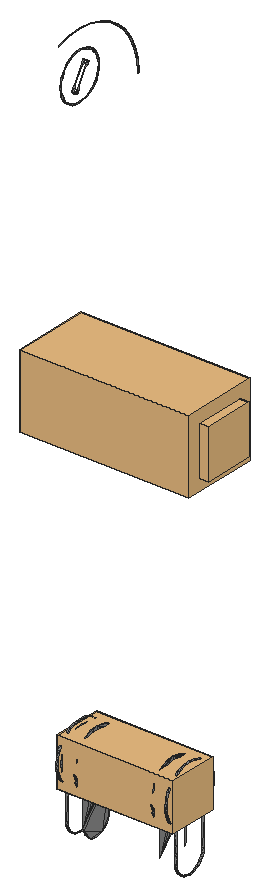
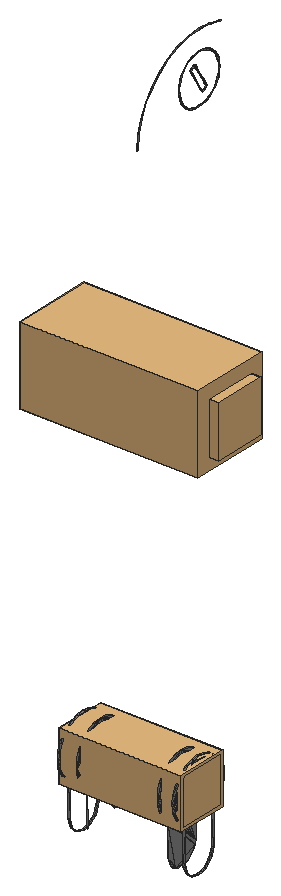
# SketchUp Ruby script. Lengths in inches.
U = 1.inch
M = Sketchup.active_model
def pt(a) = Geom::Point3d.new(a.map { |v| v * U })
def face(e, loops, mat)
  f = e.add_face(loops[0].map { |a| pt(a) })
  loops[1..].each { |l| e.add_face(l.map { |a| pt(a) }).erase! }
  f.material = f.back_material = mat if mat
  f
end
# faces: each face lists its corners as indices into pts; further lists are holes
def faces(e, pts, list, mat = nil) = list.each { |f| face(e, (f[0].is_a?(Array) ? f : [f]).map { |l| l.map { |i| pts[i] } }, mat) }
# xy, xz, yz: faces in a plane at the given z, y or x. An outline is a flat list of corners, or four numbers for a rectangle; further outlines are holes
def ring(l) = l.size == 4 ? [[l[0], l[1]], [l[2], l[1]], [l[2], l[3]], [l[0], l[3]]] : l.each_slice(2).to_a
def flat(e, list, mat, &to3) = list.each { |f| face(e, (f[0].is_a?(Array) ? f : [f]).map { |l| ring(l).map { |u, v| to3.(u, v) } }, mat) }
def xy(e, z, list, mat = nil) = flat(e, list, mat) { |x, y| [x, y, z] }
def xz(e, y, list, mat = nil) = flat(e, list, mat) { |x, z| [x, y, z] }
def yz(e, x, list, mat = nil) = flat(e, list, mat) { |y, z| [x, y, z] }
def lines(e, pts, list) = list.each { |a, b| e.add_line(pt(pts[a]), pt(pts[b])) }
# prism: a flat outline (further loops are holes) pulled along v
def prism(e, loops, v, mat = nil)
  f = face(e, loops, mat); d = Geom::Vector3d.new(v.map { |x| x * U })
  f.pushpull(f.normal.samedirection?(d) ? d.length : -d.length)
end
def box(e, o, s, mat = nil) = prism(e, [[o, [o[0] + s[0], o[1], o[2]], [o[0] + s[0], o[1] + s[1], o[2]], [o[0], o[1] + s[1], o[2]]]], [0, 0, s[2]], mat)
def at(x, y, z, deg = 0) = Geom::Transformation.translation(pt([x, y, z])) * Geom::Transformation.rotation(ORIGIN, Z_AXIS, deg.degrees)
def axes(o, x, y, z) = Geom::Transformation.new([*x, 0, *y, 0, *z, 0, *pt(o).to_a, 1])
def part(name) = M.definitions.add(name)
# library, detail: a bought-in or finely detailed component or shape, given as its bounding box
def library(name, o, s) = part(name).tap { |d| box(d.entities, o, s) }
def detail(e, o, s) = box(e.add_group.entities, o, s)
def put(e, d, t, mat = nil) = e.add_instance(d, t).tap { |i| i.material = mat if mat }
def group(e, t, mat = nil) = e.add_group.tap { |g| g.transformation = t; g.material = mat if mat }.entities
root = M.entities
M.materials.add("Material \#1").color = [140, 140, 140]
c1 = library("3DGeom~14_Defintion",[-102.17,352.37,-727.27],[204.35,204.35,1000])
c2 = library("3DGeom~1_Defintion",[-60.87,347.29,-704.08],[121.74,121.75,1000])
c3 = part("3DGeom~10_Defintion")
yz(c3.entities,-68.96,[[-797.08,-844.83,-797.08,-827.59,-922.41,-827.59],[-922.41,-844.83,-797.08,-844.83,-922.41,-827.59]],"Material \#1")
yz(c3.entities,68.97,[[-922.41,-844.83,-797.08,-827.59,-797.08,-844.83],[-922.41,-844.83,-922.41,-827.59,-797.08,-827.59],[-797.08,137.93,-922.41,155.17,-797.08,155.17],[-922.41,137.93,-922.41,155.17,-797.08,137.93]],"Material \#1")
p = [[-15.8,-989.55,-844.83],[-15.8,-989.55,-827.59],[0,-991.38,-827.59],[0,-991.38,-844.83],[15.8,-989.55,-827.59],[15.8,-989.55,-844.83],
  [-30.32,-984.36,-844.83],[-30.32,-984.36,-827.59],[30.31,-984.36,-827.59],[30.31,-984.36,-844.83],[-43.12,-976.21,-844.83],[-43.12,-976.21,-827.59],
  [43.12,-976.21,-827.59],[43.12,-976.21,-844.83],[-53.81,-965.53,-844.83],[-53.81,-965.53,-827.59],[53.8,-965.53,-827.59],[53.8,-965.53,-844.83],
  [-61.95,-952.73,-844.83],[-61.95,-952.73,-827.59],[53.8,-965.53,-827.59],[61.95,-952.73,-827.59],[61.95,-952.73,-844.83],[-67.15,-938.21,-844.83],
  [-67.15,-938.21,-827.59],[67.14,-938.21,-827.59],[67.14,-938.21,-844.83],[-68.96,-922.41,-844.83],[-68.96,-922.41,-827.59],[67.14,-938.21,-827.59],
  [68.97,-922.41,-827.59],[68.97,-922.41,-844.83],[-69.1,-794.86,-844.83],[-69.1,-794.86,-827.59],[-68.96,-797.08,-827.59],[-68.96,-797.08,-844.83],
  [68.97,-797.08,-844.83],[68.97,-797.08,-827.59],[69.11,-794.71,-827.59],[69.11,-794.71,-844.83],[-69.48,-792.73,-844.83],[-69.48,-792.73,-827.59],
  [69.53,-792.51,-827.59],[69.53,-792.51,-844.83],[-70.14,-790.6875,-844.83],[-70.14,-790.6875,-827.59],[70.24,-790.48,-827.59],[70.24,-790.48,-844.83],
  [-71.08,-788.73,-844.83],[-71.08,-788.73,-827.59],[71.22,-788.57,-827.59],[71.22,-788.57,-844.83],[-72.32,-786.86,-844.83],[-72.32,-786.86,-827.59],
  [72.47,-786.78,-827.59],[72.47,-786.78,-844.83],[-73.8,-785.17,-844.83],[-73.8,-785.17,-827.59],[74,-785.04,-827.59],[74,-785.04,-844.83],
  [-75.96,-783.21,-844.83],[-75.96,-783.21,-827.59],[74,-785.04,-827.59],[75.76,-783.39,-827.59],[75.76,-783.39,-844.83],[86.625,-772.95,-827.59],
  [86.61,-772.96,-844.83],[-86.89,-773.25,-844.83],[-86.89,-773.25,-827.59],[-75.96,-783.21,-844.83],[-96.66,-761.8,-844.83],[-96.66,-761.8,-827.59],
  [86.625,-772.95,-827.59],[86.63,-772.94,-844.83],[86.61,-772.96,-844.83],[86.625,-772.95,-827.59],[86.62,-772.95,-827.59],[86.62,-772.95,-827.59],
  [96.31,-761.375,-827.59],[96.31,-761.375,-844.83],[86.63,-772.94,-844.83],[86.625,-772.95,-827.59],[86.62,-772.95,-827.59],[-104.96,-749.18,-844.83],
  [-104.96,-749.18,-827.59],[-96.66,-761.8,-827.59],[-96.66,-761.8,-844.83],[96.31,-761.375,-827.59],[104.62,-748.77,-827.59],[104.62,-748.77,-844.83],
  [-111.64,-735.52,-844.83],[-111.64,-735.52,-827.59],[111.39,-735.21,-827.59],[111.39,-735.21,-844.83],[-116.49,-721.23,-844.83],[-116.49,-721.23,-827.59],
  [116.4375,-720.78,-827.59],[116.4375,-720.78,-844.83],[-119.64,-705.62,-844.83],[-119.64,-705.62,-827.59],[119.6,-705.57,-827.59],[119.6,-705.57,-844.83],
  [-120.6875,-689.65,-844.83],[-120.6875,-689.65,-827.59],[120.69,-689.65,-827.59],[120.69,-689.65,-844.83],[-117.5,-662,-844.83],[-117.5,-662,-827.59],
  [117.5,-662,-827.59],[117.5,-662,-844.83],[-108.41,-636.61,-844.83],[-108.41,-636.61,-827.59],[117.5,-662,-844.83],[108.41,-636.61,-827.59],
  [108.41,-636.61,-844.83],[-93.91,-613.95,-844.83],[-93.91,-613.95,-827.59],[-108.41,-636.61,-827.59],[108.41,-636.61,-844.83],[94.16,-614.19,-827.59],
  [94.16,-614.19,-844.83],[94.16,-614.19,-827.59],[75.46,-595.5,-827.59],[75.46,-595.5,-844.83],[-75.46,-595.5,-844.83],[-75.46,-595.5,-827.59],
  [-93.91,-613.95,-827.59],[-93.91,-613.95,-827.59],[-93.91,-613.95,-844.83],[-53.05,-581.24,-844.83],[-53.05,-581.24,-827.59],[-75.46,-595.5,-827.59],
  [-75.46,-595.5,-844.83],[53.05,-581.24,-827.59],[53.05,-581.24,-844.83],[-27.65,-572.16,-844.83],[-27.65,-572.16,-827.59],[-53.05,-581.24,-827.59],
  [-53.05,-581.24,-844.83],[27.66,-572.16,-827.59],[27.66,-572.16,-844.83],[0,-568.97,-844.83],[0,-568.97,-827.59],[-27.65,-572.16,-827.59],
  [-27.65,-572.16,-844.83],[0,-568.97,-844.83],[-15.8,-989.55,155.17],[0,-991.38,155.17],[0,-991.38,137.93],[-15.8,-989.55,137.93],
  [15.8,-989.55,155.17],[15.8,-989.55,137.93],[-30.32,-984.36,155.17],[-30.32,-984.36,137.93],[30.31,-984.36,155.17],[30.31,-984.36,137.93],
  [-43.125,-976.22,155.17],[-43.125,-976.22,137.93],[43.12,-976.22,155.17],[43.12,-976.22,137.93],[-53.81,-965.53,155.17],[-53.81,-965.53,137.93],
  [53.8,-965.53,155.17],[53.8,-965.53,137.93],[-61.96,-952.73,155.17],[-61.95,-952.73,137.93],[61.95,-952.73,155.17],[61.95,-952.73,137.93],
  [53.8,-965.53,137.93],[-67.15,-938.21,155.17],[-67.15,-938.21,137.93],[67.14,-938.21,155.17],[67.14,-938.21,137.93],[-68.96,-922.41,155.17],
  [-68.96,-922.41,137.93],[68.97,-922.41,155.17],[68.97,-922.41,137.93],[67.14,-938.21,137.93],[-68.97,-797.08,155.17],[-68.97,-797.08,137.93],
  [-69.1,-794.86,155.17],[-69.1,-794.86,137.93],[68.97,-797.08,155.17],[69.11,-794.71,155.17],[69.11,-794.71,137.93],[68.97,-797.08,137.93],
  [-69.48,-792.73,155.17],[-69.48,-792.73,137.93],[69.53,-792.51,155.17],[69.53,-792.51,137.93],[-70.14,-790.6875,155.17],[-70.14,-790.6875,137.93],
  [70.24,-790.48,155.17],[70.24,-790.48,137.93],[-71.08,-788.73,155.17],[-71.08,-788.73,137.93],[71.22,-788.57,155.17],[71.22,-788.57,137.93],
  [-72.32,-786.86,155.17],[-72.32,-786.86,137.93],[72.47,-786.78,155.17],[72.47,-786.78,137.93],[-73.8,-785.17,155.17],[-73.8,-785.17,137.93],
  [74,-785.04,155.17],[74,-785.04,137.93],[-75.96,-783.21,155.17],[-75.96,-783.21,137.93],[75.76,-783.39,155.17],[75.76,-783.39,137.93],
  [74,-785.04,137.93],[86.61,-772.96,155.17],[86.625,-772.95,137.93],[-86.88,-773.25,155.17],[-75.96,-783.21,155.17],[-86.88,-773.25,137.93],
  [-96.66,-761.8,155.17],[-96.66,-761.8,137.93],[86.63,-772.94,155.17],[86.625,-772.95,137.93],[86.61,-772.96,155.17],[86.62,-772.95,137.93],
  [86.625,-772.95,137.93],[96.31,-761.375,155.17],[96.31,-761.375,137.93],[86.62,-772.95,137.93],[86.63,-772.94,155.17],[86.62,-772.95,137.93],
  [86.625,-772.95,137.93],[-104.96,-749.18,155.17],[-96.66,-761.8,155.17],[-96.66,-761.8,137.93],[-104.96,-749.18,137.93],[104.62,-748.77,155.17],
  [104.62,-748.77,137.93],[96.31,-761.375,137.93],[-111.64,-735.52,155.17],[-111.64,-735.52,137.93],[111.39,-735.21,155.17],[111.39,-735.21,137.93],
  [-116.49,-721.23,155.17],[-116.49,-721.23,137.93],[116.4375,-720.78,155.17],[116.4375,-720.78,137.93],[-119.64,-705.62,155.17],[-119.64,-705.62,137.93],
  [119.6,-705.57,155.17],[119.6,-705.57,137.93],[-120.6875,-689.65,155.17],[-120.6875,-689.65,137.93],[120.69,-689.65,155.17],[120.69,-689.65,137.93],
  [-117.5,-662,155.17],[-117.5,-662,137.93],[117.5,-662,155.17],[117.5,-662,137.93],[-108.41,-636.61,155.17],[-108.41,-636.61,137.93],
  [117.5,-662,155.17],[108.41,-636.61,155.17],[108.41,-636.61,137.93],[-93.91,-613.95,155.17],[-108.41,-636.61,137.93],[-93.91,-613.95,137.93],
  [108.41,-636.61,155.17],[94.16,-614.19,155.17],[94.16,-614.19,137.93],[75.46,-595.5,155.17],[75.46,-595.5,137.93],[94.16,-614.19,137.93],
  [-75.46,-595.5,155.17],[-93.91,-613.95,155.17],[-93.91,-613.95,137.93],[-75.46,-595.5,137.93],[-53.05,-581.24,155.17],[-75.46,-595.5,155.17],
  [-75.46,-595.5,137.93],[-53.05,-581.24,137.93],[53.05,-581.24,155.17],[53.05,-581.24,137.93],[-27.65,-572.16,155.17],[-53.05,-581.24,155.17],
  [-53.05,-581.24,137.93],[-27.65,-572.16,137.93],[27.65,-572.16,155.17],[27.65,-572.16,137.93],[0,-568.97,155.17],[-27.65,-572.16,155.17],
  [-27.65,-572.16,137.93],[0,-568.97,137.93],[0,-568.97,155.17]]
faces(c3.entities,p,[[0,1,2],[2,3,0],[3,2,4],[4,5,3],[6,7,1],[1,0,6],[5,4,8],[8,9,5],
  [10,11,7],[7,6,10],[9,8,12],[12,13,9],[14,15,11],[11,10,14],[13,12,16],[16,17,13],
  [18,19,15],[15,14,18],[17,20,21],[21,22,17],[23,24,19],[19,18,23],[22,21,25],[25,26,22],
  [27,28,24],[24,23,27],[26,29,30],[30,31,26],[32,33,34],[34,35,32],[36,37,38],[38,39,36],
  [40,41,33],[33,32,40],[39,38,42],[42,43,39],[44,45,41],[41,40,44],[43,42,46],[46,47,43],
  [48,49,45],[45,44,48],[47,46,50],[50,51,47],[52,53,49],[49,48,52],[51,50,54],[54,55,51],
  [56,57,53],[53,52,56],[55,54,58],[58,59,55],[60,61,57],[57,56,60],[59,62,63],[63,64,59],
  [64,63,65],[65,66,64],[67,68,61],[61,69,67],[70,71,68],[68,67,70],[72,73,66],[74,75,76],
  [73,77,78],[78,79,73],[80,81,82],[83,84,85],[85,86,83],[79,87,88],[88,89,79],[90,91,84],
  [84,83,90],[89,88,92],[92,93,89],[94,95,91],[91,90,94],[93,92,96],[96,97,93],[98,99,95],
  [95,94,98],[97,96,100],[100,101,97],[102,103,99],[99,98,102],[101,100,104],[104,105,101],[106,107,103],
  [103,102,106],[105,104,108],[108,109,105],[110,111,107],[107,106,110],[112,108,113],[113,114,112],[115,116,117],
  [117,110,115],[118,113,119],[119,120,118],[120,121,122],[122,123,120],[124,125,126],[127,128,124],[129,130,131],
  [131,132,129],[123,122,133],[133,134,123],[135,136,137],[137,138,135],[134,133,139],[139,140,134],[141,142,143],
  [143,144,141],[140,139,142],[142,145,140],[146,147,148],[148,149,146],[147,150,151],[151,148,147],[152,146,149],
  [149,153,152],[150,154,155],[155,151,150],[156,152,153],[153,157,156],[154,158,159],[159,155,154],[160,156,157],
  [157,161,160],[158,162,163],[163,159,158],[164,160,161],[161,165,164],[162,166,167],[167,168,162],[169,164,165],
  [165,170,169],[166,171,172],[172,167,166],[173,169,170],[170,174,173],[171,175,176],[176,177,171],[178,173,174],
  [174,179,178],[180,178,179],[179,181,180],[182,183,184],[184,185,182],[186,180,181],[181,187,186],[183,188,189],
  [189,184,183],[190,186,187],[187,191,190],[188,192,193],[193,189,188],[194,190,191],[191,195,194],[192,196,197],
  [197,193,192],[198,194,195],[195,199,198],[196,200,201],[201,197,196],[202,198,199],[199,203,202],[200,204,205],
  [205,201,200],[206,202,203],[203,207,206],[204,208,209],[209,210,204],[208,211,212],[212,209,208],[213,214,207],
  [207,215,213],[216,213,215],[215,217,216],[211,218,219],[220,221,222],[218,223,224],[224,225,218],[226,227,228],
  [229,230,231],[231,232,229],[223,233,234],[234,235,223],[236,229,232],[232,237,236],[233,238,239],[239,234,233],
  [240,236,237],[237,241,240],[238,242,243],[243,239,238],[244,240,241],[241,245,244],[242,246,247],[247,243,242],
  [248,244,245],[245,249,248],[246,250,251],[251,247,246],[252,248,249],[249,253,252],[250,254,255],[255,251,250],
  [256,252,253],[253,257,256],[258,259,260],[260,255,258],[261,256,262],[262,263,261],[264,265,266],[266,260,264],
  [265,267,268],[268,269,265],[270,271,272],[272,273,270],[274,275,276],[276,277,274],[267,278,279],[279,268,267],
  [280,281,282],[282,283,280],[278,284,285],[285,279,278],[286,287,288],[288,289,286],[284,290,289],[289,285,284]],"Material \#1")
c4 = library("3DGeom~12_Defintion",[-95.68,-755.75,-830.03],[191.36,191.37,1000])
c5 = library("3DGeom~13_Defintion",[-84.91,-744.98,-830.03],[169.82,169.83,1000])
xy(root,47.143,[[362.669,397.987,362.669,398.031,362.882,397.987],[362.882,397.987,362.669,398.031,362.882,398.031]],"Material \#1")
xy(root,47.538,[[362.669,397.98,362.882,397.98,362.882,398.053],[362.669,397.98,362.882,398.053,362.669,398.053]],"Material \#1")
xz(root,397.976,[[362.669,47.314,362.882,47.314,362.882,47.342],[362.669,47.314,362.882,47.342,362.669,47.342]],"Material \#1")
xz(root,397.98,[[362.669,47.39,362.882,47.39,362.882,47.454]],"Material \#1")
xz(root,397.987,[[362.669,47.252,362.882,47.252,362.882,47.286],[362.669,47.252,362.882,47.286,362.669,47.286]],"Material \#1")
xz(root,398.046,[[362.882,47.215,362.669,47.252,362.882,47.252]],"Material \#1")
xz(root,398.053,[[362.882,47.473,362.669,47.538,362.882,47.538]],"Material \#1")
yz(root,362.698,[[398.888,54.238,398.888,54.399,398.873,54.397],[398.888,54.238,398.903,54.239,398.888,54.399],[398.017,54.303,397.967,54.322,397.964,54.307],[398.017,54.303,398.017,54.318,397.967,54.322],[398.017,54.303,398.069,54.307,398.017,54.318],
  [397.964,54.307,397.92,54.335,397.914,54.321],[397.964,54.307,397.967,54.322,397.92,54.335],[398.069,54.307,398.067,54.322,398.017,54.318],[398.069,54.307,398.119,54.321,398.067,54.322],[397.914,54.321,397.876,54.355,397.868,54.342],
  [397.914,54.321,397.92,54.335,397.876,54.355],[398.119,54.321,398.114,54.335,398.067,54.322],[398.119,54.321,398.165,54.342,398.114,54.335],[398.114,54.335,398.165,54.342,398.158,54.355],[397.868,54.342,397.837,54.382,397.827,54.37],
  [397.868,54.342,397.876,54.355,397.837,54.382],[398.165,54.342,398.206,54.37,398.158,54.355],[398.158,54.355,398.206,54.37,398.197,54.382],[397.827,54.37,397.803,54.414,397.792,54.405],[397.827,54.37,397.837,54.382,397.803,54.414],
  [398.206,54.37,398.242,54.405,398.197,54.382],[398.197,54.382,398.242,54.405,398.23,54.414],[398.873,54.397,398.847,54.545,398.833,54.54],[398.873,54.397,398.888,54.399,398.847,54.545],[397.792,54.405,397.776,54.452,397.763,54.445],
  [397.792,54.405,397.803,54.414,397.776,54.452],[398.242,54.405,398.271,54.445,398.23,54.414],[398.23,54.414,398.271,54.445,398.258,54.452],[397.763,54.445,397.755,54.495,397.741,54.489],[397.763,54.445,397.776,54.452,397.755,54.495],
  [398.271,54.445,398.293,54.489,398.258,54.452],[398.258,54.452,398.293,54.489,398.278,54.495],[397.741,54.489,397.742,54.541,397.727,54.538],[397.741,54.489,397.755,54.495,397.742,54.541],[398.293,54.489,398.306,54.538,398.278,54.495],
  [398.278,54.495,398.306,54.538,398.291,54.541],[397.727,54.538,397.738,54.589,397.723,54.589],[397.727,54.538,397.742,54.541,397.738,54.589],[398.306,54.538,398.311,54.603,398.291,54.541],[398.833,54.54,398.781,54.679,398.768,54.672],
  [398.833,54.54,398.847,54.545,398.781,54.679],[398.291,54.541,398.311,54.603,398.296,54.602],[397.723,54.589,397.738,54.589,397.742,54.638],[397.723,54.589,397.742,54.638,397.727,54.641],[398.296,54.602,398.306,54.641,398.291,54.638],
  [398.296,54.602,398.311,54.603,398.306,54.641],[397.742,54.638,397.755,54.684,397.727,54.641],[398.291,54.638,398.293,54.689,398.278,54.684],[398.291,54.638,398.306,54.641,398.293,54.689],[397.727,54.641,397.755,54.684,397.741,54.689],
  [398.768,54.672,398.69,54.804,398.679,54.794],[398.768,54.672,398.781,54.679,398.69,54.804],[397.755,54.684,397.776,54.726,397.741,54.689],[398.278,54.684,398.271,54.734,398.258,54.726],[398.278,54.684,398.293,54.689,398.271,54.734],
  [397.741,54.689,397.776,54.726,397.763,54.734],[397.776,54.726,397.803,54.764,397.763,54.734],[398.258,54.726,398.242,54.774,398.23,54.764],[398.258,54.726,398.271,54.734,398.242,54.774],[397.763,54.734,397.803,54.764,397.792,54.774],
  [397.803,54.764,397.837,54.797,397.792,54.774],[398.23,54.764,398.206,54.808,398.197,54.797],[398.23,54.764,398.242,54.774,398.206,54.808],[397.792,54.774,397.837,54.797,397.827,54.808],[398.679,54.794,398.587,54.904,398.577,54.892],
  [398.679,54.794,398.69,54.804,398.587,54.904],[397.837,54.797,397.876,54.824,397.827,54.808],[398.197,54.797,398.165,54.837,398.158,54.824],[398.197,54.797,398.206,54.808,398.165,54.837],[397.827,54.808,397.876,54.824,397.868,54.837],
  [397.876,54.824,397.92,54.844,397.868,54.837],[398.158,54.824,398.119,54.858,398.114,54.844],[398.158,54.824,398.165,54.837,398.119,54.858],[397.868,54.837,397.92,54.844,397.914,54.858],[397.92,54.844,397.967,54.857,397.914,54.858],
  [398.114,54.844,398.069,54.871,398.067,54.857],[398.114,54.844,398.119,54.858,398.069,54.871],[397.967,54.857,397.964,54.871,397.914,54.858],[397.967,54.857,398.017,54.861,397.964,54.871],[398.067,54.857,398.017,54.876,398.017,54.861],
  [398.067,54.857,398.069,54.871,398.017,54.876],[398.017,54.861,398.017,54.876,397.964,54.871],[398.577,54.892,398.464,54.989,398.456,54.976],[398.577,54.892,398.587,54.904,398.464,54.989],[398.456,54.976,398.326,55.053,398.32,55.039],
  [398.456,54.976,398.464,54.989,398.326,55.053],[397.713,55.039,397.86,55.078,397.708,55.053],[398.32,55.039,398.176,55.093,398.173,55.078],[398.32,55.039,398.326,55.053,398.176,55.093],[397.708,55.053,397.86,55.078,397.857,55.093],
  [397.86,55.078,398.017,55.092,397.857,55.093],[398.173,55.078,398.017,55.107,398.017,55.092],[398.173,55.078,398.176,55.093,398.017,55.107],[398.017,55.092,398.017,55.107,397.857,55.093]],"Material \#1")
yz(root,362.721,[[398.017,47.044,397.941,47.064,397.938,47.055],[398.017,47.044,398.017,47.054,397.941,47.064],[398.017,47.044,398.095,47.055,398.017,47.054],[398.017,47.054,398.095,47.055,398.093,47.064],[397.938,47.055,397.87,47.093,397.865,47.084],
  [397.938,47.055,397.941,47.064,397.87,47.093],[398.095,47.055,398.169,47.084,398.093,47.064],[398.093,47.064,398.169,47.084,398.164,47.093],[397.865,47.084,397.809,47.138,397.802,47.131],[397.865,47.084,397.87,47.093,397.809,47.138],
  [398.169,47.084,398.232,47.131,398.164,47.093],[398.164,47.093,398.232,47.131,398.224,47.138],[397.802,47.131,397.763,47.197,397.754,47.192],[397.802,47.131,397.809,47.138,397.763,47.197],[398.232,47.131,398.28,47.192,398.224,47.138],
  [398.224,47.138,398.28,47.192,398.271,47.197],[397.754,47.192,397.733,47.266,397.723,47.264],[397.754,47.192,397.763,47.197,397.733,47.266],[398.28,47.192,398.31,47.264,398.271,47.197],[398.271,47.197,398.31,47.264,398.3,47.266],
  [397.723,47.264,397.723,47.34,397.713,47.34],[397.723,47.264,397.733,47.266,397.723,47.34],[398.31,47.264,398.321,47.34,398.3,47.266],[398.3,47.266,398.321,47.34,398.31,47.34],[397.713,47.34,397.723,47.34,397.733,47.414],
  [397.713,47.34,397.733,47.414,397.723,47.417],[398.31,47.34,398.31,47.417,398.3,47.414],[398.31,47.34,398.321,47.34,398.31,47.417],[397.733,47.414,397.763,47.483,397.723,47.417],[398.3,47.414,398.28,47.488,398.271,47.483],
  [398.3,47.414,398.31,47.417,398.28,47.488],[397.723,47.417,397.763,47.483,397.754,47.488],[397.763,47.483,397.809,47.542,397.754,47.488],[398.271,47.483,398.232,47.55,398.224,47.542],[398.271,47.483,398.28,47.488,398.232,47.55],
  [397.754,47.488,397.809,47.542,397.802,47.55],[397.809,47.542,397.87,47.588,397.802,47.55],[398.224,47.542,398.169,47.597,398.164,47.588],[398.224,47.542,398.232,47.55,398.169,47.597],[397.802,47.55,397.87,47.588,397.865,47.597],
  [397.87,47.588,397.941,47.617,397.865,47.597],[398.164,47.588,398.095,47.626,398.093,47.617],[398.164,47.588,398.169,47.597,398.095,47.626],[397.865,47.597,397.941,47.617,397.938,47.626],[397.941,47.617,398.017,47.626,397.938,47.626],
  [398.093,47.617,398.017,47.636,398.017,47.626],[398.093,47.617,398.095,47.626,398.017,47.636],[397.938,47.626,398.017,47.626,398.017,47.636]],"Material \#1")
yz(root,362.882,[[397.987,47.143,398.031,47.143,398.002,47.173],[398.031,47.143,398.046,47.173,398.002,47.173],[398.002,47.173,398.046,47.173,397.994,47.183],[398.046,47.173,398.053,47.183,397.994,47.183],[397.994,47.183,398.053,47.183,397.994,47.205],
  [398.053,47.183,398.053,47.205,397.994,47.205],[397.994,47.205,398.053,47.205,398.002,47.215],[398.053,47.205,398.046,47.215,398.002,47.215],[398.002,47.215,398.046,47.215,397.987,47.252],[398.046,47.215,398.046,47.252,397.987,47.252],
  [397.987,47.252,398.046,47.252,397.987,47.286],[398.046,47.252,398.046,47.286,397.987,47.286],[397.987,47.286,398.046,47.286,397.976,47.314],[398.046,47.286,398.057,47.314,397.976,47.314],[397.976,47.314,398.057,47.314,397.976,47.342],
  [398.057,47.314,398.057,47.342,397.976,47.342],[397.976,47.342,398.057,47.342,397.987,47.37],[398.057,47.342,398.046,47.37,397.987,47.37],[397.987,47.37,398.046,47.37,397.98,47.39],[398.046,47.37,398.053,47.39,397.98,47.39],
  [397.98,47.39,398.053,47.39,397.98,47.454],[398.053,47.39,398.053,47.454,397.98,47.454],[397.98,47.454,398.053,47.454,397.989,47.459],[398.053,47.454,398.044,47.459,397.989,47.459],[397.989,47.459,398.044,47.459,397.989,47.469],
  [398.044,47.459,398.044,47.469,397.989,47.469],[397.989,47.469,398.044,47.469,397.98,47.473],[398.044,47.469,398.053,47.473,397.98,47.473],[397.98,47.473,398.053,47.473,397.98,47.538],[398.053,47.473,398.053,47.538,397.98,47.538]],"Material \#1")
yz(root,362.905,[[398.017,46.487,397.932,46.506,398.101,46.506],[398.017,46.487,397.973,46.492,397.932,46.506],[398.017,46.487,398.101,46.506,398.061,46.492],[397.932,46.506,397.829,46.632,398.101,46.506],[397.932,46.506,397.867,46.557,397.829,46.632],
  [398.101,46.506,397.829,46.632,398.209,47.033],[397.932,46.506,397.896,46.528,397.867,46.557],[398.101,46.506,398.167,46.557,398.137,46.528],[398.101,46.506,398.204,46.632,398.167,46.557],[398.101,46.506,398.209,47.033,398.204,46.632],
  [397.867,46.557,397.844,46.592,397.829,46.632],[398.167,46.557,398.204,46.632,398.19,46.592],[397.829,46.632,397.824,46.675,398.217,47.062],[397.829,46.632,398.21,47.041,398.209,47.033],[397.829,46.632,398.211,47.048,398.21,47.041],
  [397.829,46.632,398.213,47.055,398.211,47.048],[397.829,46.632,398.217,47.062,398.213,47.055],[398.204,46.632,398.209,47.033,398.209,46.675],[397.824,46.675,397.824,47.033,397.947,47.052],[397.824,46.675,397.947,47.052,398.017,47.044],
  [397.824,46.675,398.017,47.044,398.086,47.052],[397.824,46.675,398.086,47.052,398.15,47.075],[397.824,46.675,398.15,47.075,398.207,47.109],[397.824,46.675,398.207,47.109,398.254,47.155],[397.824,46.675,398.254,47.155,398.217,47.062],
  [397.824,47.033,397.822,47.049,397.947,47.052],[397.824,47.033,397.824,47.041,397.822,47.049],[397.822,47.049,397.817,47.062,397.947,47.052],[397.822,47.049,397.82,47.056,397.817,47.062],[397.947,47.052,397.817,47.062,397.883,47.075],
  [397.817,47.062,397.676,47.296,397.78,47.155],[397.817,47.062,397.812,47.068,397.676,47.296],[397.817,47.062,397.78,47.155,397.827,47.109],[397.817,47.062,397.827,47.109,397.883,47.075],[398.217,47.062,398.254,47.155,398.29,47.21],
  [398.217,47.062,398.29,47.21,398.358,47.296],[398.217,47.062,398.358,47.296,398.221,47.068],[397.812,47.068,397.807,47.074,397.676,47.296],[398.221,47.068,398.358,47.296,398.226,47.074],[397.807,47.074,397.742,47.141,397.676,47.296],
  [397.807,47.074,397.801,47.08,397.742,47.141],[398.226,47.074,398.293,47.14,398.233,47.08],[398.226,47.074,398.358,47.296,398.293,47.14],[397.801,47.08,397.77,47.109,397.742,47.141],[398.233,47.08,398.293,47.14,398.265,47.108],
  [398.293,47.14,398.335,47.213,398.316,47.175],[398.293,47.14,398.358,47.296,398.335,47.213],[397.742,47.141,397.718,47.176,397.699,47.214],[397.78,47.155,397.676,47.296,397.744,47.21],[398.29,47.21,398.3125,47.273,398.358,47.296],
  [398.335,47.213,398.358,47.296,398.349,47.253],[398.3125,47.273,398.321,47.34,398.358,47.296],[398.358,47.296,398.285,47.55,398.352,47.417],[398.358,47.296,398.29,47.47,398.285,47.55],[398.358,47.296,398.3125,47.408,398.29,47.47],
  [398.358,47.296,398.321,47.34,398.3125,47.408],[398.358,47.296,398.352,47.417,398.361,47.34],[397.721,47.408,397.748,47.55,397.744,47.47],[398.352,47.417,398.285,47.55,398.326,47.488],[397.744,47.47,397.748,47.55,397.78,47.525],
  [398.29,47.47,398.254,47.525,398.285,47.55],[397.78,47.525,397.748,47.55,397.827,47.571],[398.254,47.525,398.207,47.571,398.285,47.55],[397.748,47.55,397.802,47.602,397.865,47.642],[397.748,47.55,397.865,47.642,398.017,47.676],
  [397.748,47.55,397.883,47.606,397.827,47.571],[397.748,47.55,398.017,47.676,397.883,47.606],[398.285,47.55,398.017,47.676,398.168,47.642],[398.285,47.55,398.15,47.606,398.017,47.676],[398.285,47.55,398.207,47.571,398.15,47.606],
  [398.285,47.55,398.168,47.642,398.232,47.602],[397.883,47.606,398.017,47.676,397.947,47.628],[398.15,47.606,398.086,47.628,398.017,47.676],[397.947,47.628,398.017,47.676,398.017,47.636],[398.086,47.628,398.017,47.636,398.017,47.676],
  [397.865,47.642,397.938,47.667,398.017,47.676],[398.168,47.642,398.017,47.676,398.096,47.667]],"Material \#1")
yz(root,363.822,[[398.204,46.632,398.209,46.675,398.209,47.033],[397.824,46.675,397.947,47.052,397.824,47.033],[397.824,46.675,398.017,47.044,397.947,47.052],[397.824,46.675,398.086,47.052,398.017,47.044],[397.824,46.675,398.254,47.155,398.207,47.109],
  [397.824,47.033,397.947,47.052,397.822,47.049],[397.822,47.049,397.947,47.052,397.817,47.062],[397.947,47.052,397.883,47.075,397.817,47.062],[397.817,47.062,397.676,47.296,397.812,47.068],[397.817,47.062,397.78,47.155,397.676,47.296],
  [397.817,47.062,397.883,47.075,397.827,47.109],[398.217,47.062,398.221,47.068,398.358,47.296],[397.812,47.068,397.676,47.296,397.807,47.074],[398.221,47.068,398.226,47.074,398.358,47.296],[397.807,47.074,397.676,47.296,397.742,47.141],
  [397.807,47.074,397.742,47.141,397.801,47.08],[397.801,47.08,397.742,47.141,397.77,47.109],[397.742,47.141,397.699,47.214,397.718,47.176],[397.78,47.155,397.744,47.21,397.676,47.296],[398.335,47.213,398.349,47.253,398.358,47.296],
  [398.358,47.296,398.285,47.55,398.29,47.47],[398.358,47.296,398.352,47.417,398.285,47.55],[398.358,47.296,398.29,47.47,398.3125,47.408],[398.358,47.296,398.3125,47.408,398.321,47.34],[398.358,47.296,398.361,47.34,398.352,47.417],
  [397.721,47.408,397.744,47.47,397.748,47.55],[398.352,47.417,398.326,47.488,398.285,47.55],[397.744,47.47,397.78,47.525,397.748,47.55],[398.29,47.47,398.285,47.55,398.254,47.525],[397.78,47.525,397.827,47.571,397.748,47.55],
  [398.254,47.525,398.285,47.55,398.207,47.571],[397.748,47.55,397.827,47.571,397.883,47.606],[397.748,47.55,397.865,47.642,397.802,47.602],[397.748,47.55,397.883,47.606,398.017,47.676],[397.748,47.55,398.017,47.676,397.865,47.642],
  [398.285,47.55,398.017,47.676,398.15,47.606],[398.285,47.55,398.168,47.642,398.017,47.676],[398.285,47.55,398.15,47.606,398.207,47.571],[398.285,47.55,398.232,47.602,398.168,47.642],[397.883,47.606,397.947,47.628,398.017,47.676],
  [398.15,47.606,398.017,47.676,398.086,47.628],[397.947,47.628,398.017,47.636,398.017,47.676],[398.086,47.628,398.017,47.676,398.017,47.636],[397.865,47.642,398.017,47.676,397.938,47.667],[398.168,47.642,398.096,47.667,398.017,47.676]],"Material \#1")
p = [[362.882,398.002,47.173],[362.669,397.998,47.178],[362.669,397.987,47.143],[362.669,397.987,47.143],[362.882,397.987,47.143],[362.882,398.002,47.173],
  [362.669,398.05,47.178],[362.882,398.046,47.173],[362.882,398.031,47.143],[362.669,398.031,47.143],[362.669,398.05,47.178],[362.882,398.046,47.215],
  [362.669,398.05,47.21],[362.669,398.046,47.252],[362.882,397.987,47.252],[362.669,397.987,47.252],[362.669,397.998,47.21],[362.669,398.05,47.21],
  [362.882,398.053,47.205],[362.882,398.053,47.183],[362.669,398.05,47.178],[362.669,397.998,47.178],[362.882,397.994,47.183],[362.882,397.994,47.205],
  [362.669,397.998,47.21],[362.669,398.05,47.21],[362.882,398.046,47.215],[362.882,398.053,47.205],[362.669,398.05,47.178],[362.882,398.053,47.183],
  [362.882,398.046,47.173],[362.669,397.998,47.21],[362.882,398.002,47.215],[362.882,397.987,47.252],[362.669,397.998,47.21],[362.882,397.994,47.205],
  [362.882,398.002,47.215],[362.669,397.998,47.178],[362.882,398.002,47.173],[362.882,397.994,47.183],[362.882,398.046,47.286],[362.669,398.051,47.3],
  [362.669,398.057,47.328],[362.882,398.046,47.252],[362.669,398.046,47.252],[362.669,398.051,47.3],[362.882,397.987,47.37],[362.669,397.987,47.37],
  [362.669,397.976,47.342],[362.882,397.976,47.314],[362.669,397.976,47.314],[362.669,397.987,47.286],[362.882,398.057,47.342],[362.669,398.051,47.356],
  [362.669,398.049,47.38],[362.669,398.057,47.328],[362.882,398.057,47.314],[362.882,398.046,47.286],[362.669,398.051,47.3],[362.882,398.046,47.286],
  [362.882,398.046,47.252],[362.669,397.976,47.342],[362.882,397.976,47.342],[362.882,397.987,47.37],[362.669,397.987,47.286],[362.882,397.987,47.286],
  [362.882,397.976,47.314],[362.669,398.049,47.38],[362.882,398.046,47.37],[362.882,398.057,47.342],[362.882,398.057,47.314],[362.669,398.057,47.328],
  [362.669,398.051,47.356],[362.669,398.051,47.356],[362.882,398.057,47.342],[362.882,398.057,47.314],[362.882,397.98,47.454],[362.669,397.984,47.466],
  [362.669,397.98,47.39],[362.882,397.98,47.39],[362.669,397.98,47.39],[362.669,397.987,47.37],[362.882,398.053,47.39],[362.669,398.053,47.394],
  [362.669,398.05,47.459],[362.882,398.046,47.37],[362.669,398.049,47.38],[362.669,398.053,47.394],[362.669,397.987,47.37],[362.882,397.987,47.37],
  [362.882,397.98,47.39],[362.669,398.05,47.459],[362.882,398.053,47.454],[362.882,398.053,47.39],[362.669,398.053,47.394],[362.882,398.053,47.39],
  [362.882,398.046,47.37],[362.882,397.98,47.538],[362.669,397.98,47.538],[362.669,397.984,47.466],[362.882,398.053,47.473],[362.669,398.05,47.459],
  [362.669,398.053,47.538],[362.669,397.984,47.466],[362.882,397.98,47.473],[362.882,397.98,47.538],[362.669,397.984,47.466],[362.882,397.98,47.454],
  [362.882,397.989,47.459],[362.669,398.05,47.459],[362.882,398.044,47.469],[362.882,398.044,47.459],[362.669,398.05,47.459],[362.882,398.053,47.473],
  [362.669,398.05,47.459],[362.882,398.053,47.454],[362.669,397.984,47.466],[362.882,397.989,47.469],[362.882,397.98,47.473],[362.669,397.984,47.466],
  [362.703,397.963,54.432],[362.722,397.963,54.432],[362.722,397.931,54.445],[362.703,397.931,54.445],[362.722,397.903,54.466],[362.703,397.903,54.466],
  [362.698,397.982,54.465],[362.716,397.982,54.465],[362.716,397.923,54.498],[362.698,397.923,54.498],[362.715,397.94,54.527],[362.696,397.94,54.527],
  [362.715,398.034,54.685],[362.696,398.034,54.685],[362.696,398.093,54.652],[362.715,398.093,54.652],[362.715,398,54.494],[362.696,398,54.494],
  [362.716,398.051,54.714],[362.698,398.051,54.714],[362.722,398.07,54.747],[362.703,398.07,54.747],[362.722,398.102,54.734],[362.703,398.102,54.734],
  [362.722,398.13,54.713],[362.703,398.13,54.713],[362.716,398.111,54.681],[362.698,398.111,54.681]]
faces(root,p,[[0,1,2],[3,4,5],[6,7,8],[8,9,10],[11,12,13],[14,15,16],[17,18,19],[19,20,17],
  [21,22,23],[23,24,21],[25,26,27],[28,29,30],[31,32,33],[34,35,36],[37,38,39],[40,41,42],
  [43,44,45],[46,47,48],[49,50,51],[52,53,54],[55,56,57],[58,59,60],[61,62,63],[64,65,66],
  [67,68,69],[70,71,72],[73,74,75],[76,77,78],[79,80,81],[82,83,84],[85,86,87],[88,89,90],
  [91,92,93],[94,95,96],[97,98,99],[100,101,102],[103,104,105],[106,107,108],[109,110,111],[112,113,110],
  [114,111,115],[116,117,118],[119,108,117],[120,121,122],[122,123,120],[123,122,124],[124,125,123],[126,127,121],
  [121,120,126],[125,124,128],[128,129,125],[129,128,130],[130,131,129],[131,130,132],[132,133,131],[134,135,136],
  [136,137,134],[137,136,127],[127,126,137],[133,132,138],[138,139,133],[139,138,140],[140,141,139],[141,140,142],
  [142,143,141],[143,142,144],[144,145,143],[145,144,146],[146,147,145],[147,146,135],[135,134,147]],"Material \#1")
put(root,c1,axes([363.82,398.02,49.3125],[0,-0.00446,0],[0,0,0.00434],[0.00202,0,0]),"Material \#1")
put(root,c2,axes([363.82,398.02,49.3125],[0,-0.00496,0],[0,0,0.00483],[0.00225,0,0]),"Material \#1")
put(root,c3,axes([363.82,398.02,49.3125],[0,-0.00294,0],[0,0,0.00286],[0.00133,0,0]),"Material \#1")
put(root,c4,axes([363.82,398.02,49.3125],[0,-0.00307,0],[0,0,0.00299],[0.00139,0,0]),"Material \#1")
put(root,c5,axes([363.82,398.02,49.3125],[0,-0.00307,0],[0,0,0.00299],[0.00139,0,0]),"Material \#1")
